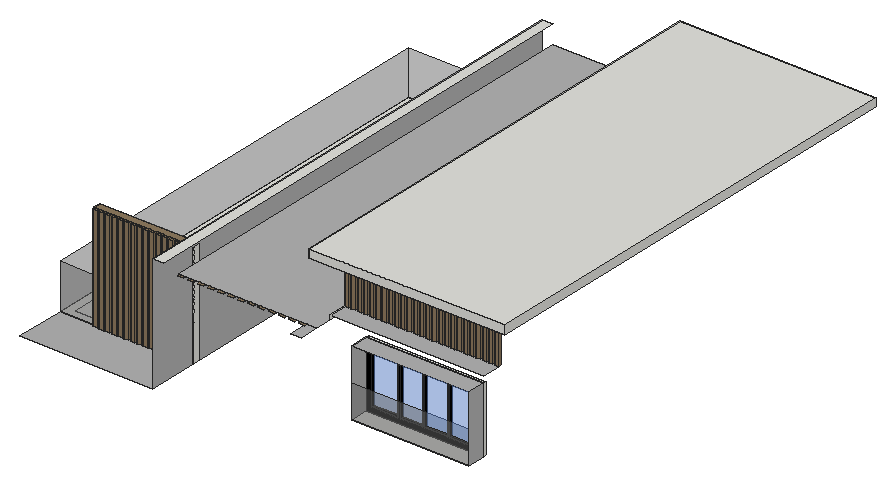
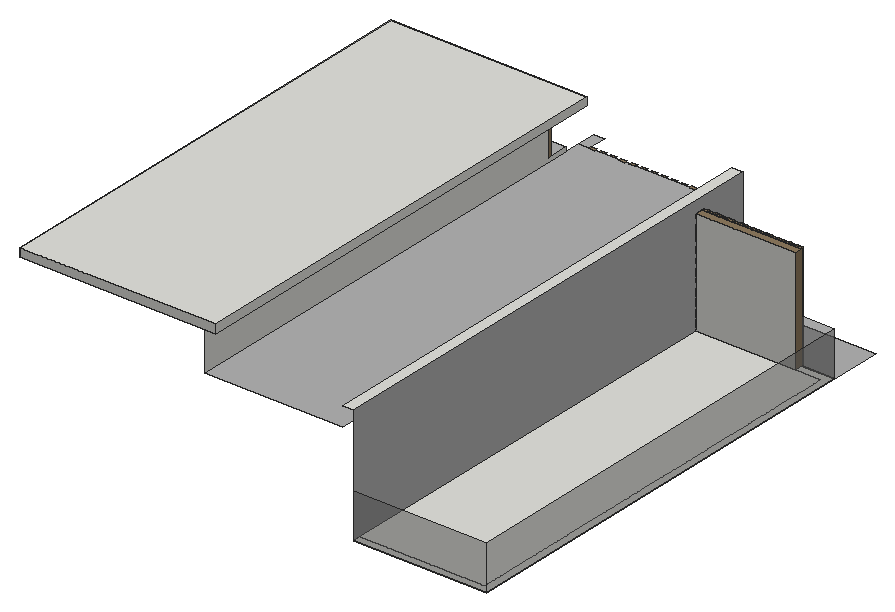
# SketchUp Ruby script. Lengths in inches.
U = 1.inch
M = Sketchup.active_model
def pt(a) = Geom::Point3d.new(a.map { |v| v * U })
def face(e, loops, mat)
  f = e.add_face(loops[0].map { |a| pt(a) })
  loops[1..].each { |l| e.add_face(l.map { |a| pt(a) }).erase! }
  f.material = f.back_material = mat if mat
  f
end
# faces: each face lists its corners as indices into pts; further lists are holes
def faces(e, pts, list, mat = nil) = list.each { |f| face(e, (f[0].is_a?(Array) ? f : [f]).map { |l| l.map { |i| pts[i] } }, mat) }
# xy, xz, yz: faces in a plane at the given z, y or x. An outline is a flat list of corners, or four numbers for a rectangle; further outlines are holes
def ring(l) = l.size == 4 ? [[l[0], l[1]], [l[2], l[1]], [l[2], l[3]], [l[0], l[3]]] : l.each_slice(2).to_a
def flat(e, list, mat, &to3) = list.each { |f| face(e, (f[0].is_a?(Array) ? f : [f]).map { |l| ring(l).map { |u, v| to3.(u, v) } }, mat) }
def xy(e, z, list, mat = nil) = flat(e, list, mat) { |x, y| [x, y, z] }
def xz(e, y, list, mat = nil) = flat(e, list, mat) { |x, z| [x, y, z] }
def yz(e, x, list, mat = nil) = flat(e, list, mat) { |y, z| [x, y, z] }
def lines(e, pts, list) = list.each { |a, b| e.add_line(pt(pts[a]), pt(pts[b])) }
# prism: a flat outline (further loops are holes) pulled along v
def prism(e, loops, v, mat = nil)
  f = face(e, loops, mat); d = Geom::Vector3d.new(v.map { |x| x * U })
  f.pushpull(f.normal.samedirection?(d) ? d.length : -d.length)
end
def box(e, o, s, mat = nil) = prism(e, [[o, [o[0] + s[0], o[1], o[2]], [o[0] + s[0], o[1] + s[1], o[2]], [o[0], o[1] + s[1], o[2]]]], [0, 0, s[2]], mat)
def at(x, y, z, deg = 0) = Geom::Transformation.translation(pt([x, y, z])) * Geom::Transformation.rotation(ORIGIN, Z_AXIS, deg.degrees)
def axes(o, x, y, z) = Geom::Transformation.new([*x, 0, *y, 0, *z, 0, *pt(o).to_a, 1])
def part(name) = M.definitions.add(name)
# library, detail: a bought-in or finely detailed component or shape, given as its bounding box
def library(name, o, s) = part(name).tap { |d| box(d.entities, o, s) }
def detail(e, o, s) = box(e.add_group.entities, o, s)
def put(e, d, t, mat = nil) = e.add_instance(d, t).tap { |i| i.material = mat if mat }
def group(e, t, mat = nil) = e.add_group.tap { |g| g.transformation = t; g.material = mat if mat }.entities
root = M.entities
M.materials.add("Niraj_Hair_Gray").color = [178, 178, 178]
M.materials.add("[0035_Tan]").color = [142, 122, 95]
M.materials.add("[0137_Black]").color = [0, 0, 0]
M.materials.add("[Translucent Glass Blue]").color = [100, 149, 237]
M.materials["[Translucent Glass Blue]"].alpha = 0.5
M.materials.add("[Translucent Glass Gray]").color = [128, 128, 128]
M.materials["[Translucent Glass Gray]"].alpha = 0.5
xy(root,261.125,[[39.27,322.73,44.8,325.73],[46.45,322.73,51.99,325.73],[53.64,322.73,59.17,325.73],[60.83,322.73,66.36,325.73],[68.02,322.73,73.55,325.73],
  [75.2,322.73,80.74,325.73],[82.39,322.73,87.92,325.73],[89.58,322.73,95.11,325.73],[96.77,322.73,102.3,325.73],[103.95,322.73,109.49,325.73],
  [111.14,322.73,116.67,325.73],[118.33,322.73,123.86,325.73],[125.52,322.73,131.05,325.73],[132.7,322.73,138.24,325.73],[139.89,322.73,145.42,325.73],
  [147.08,322.73,152.61,325.73],[0,325.73,38.3125,325.73,38.3125,334.73,9,334.73,9,814.73,151.88,814.73,151.88,823.73,0,823.73],[38.3125,325.73,152.61,334.73],[9,334.73,152.61,334.73,152.61,823.73,151.88,823.73,151.88,814.73,9,814.73]])
xy(root,261.125,[[0,267.73,152.61,267.73,152.61,322.73,147.08,322.73,147.08,325.73,145.42,325.73,145.42,322.73,139.89,322.73,139.89,325.73,138.24,325.73,138.24,322.73,132.7,322.73,132.7,325.73,131.05,325.73,131.05,322.73,125.52,322.73,125.52,325.73,123.86,325.73,123.86,322.73,118.33,322.73,118.33,325.73,116.67,325.73,116.67,322.73,111.14,322.73,111.14,325.73,109.49,325.73,109.49,322.73,103.95,322.73,103.95,325.73,102.3,325.73,102.3,322.73,96.77,322.73,96.77,325.73,95.11,325.73,95.11,322.73,89.58,322.73,89.58,325.73,87.92,325.73,87.92,322.73,82.39,322.73,82.39,325.73,80.74,325.73,80.74,322.73,75.2,322.73,75.2,325.73,73.55,325.73,73.55,322.73,68.02,322.73,68.02,325.73,66.36,325.73,66.36,322.73,60.83,322.73,60.83,325.73,59.17,325.73,59.17,322.73,53.64,322.73,53.64,325.73,51.99,325.73,51.99,322.73,46.45,322.73,46.45,325.73,44.8,325.73,44.8,322.73,39.27,322.73,39.27,325.73,0,325.73]],"Niraj_Hair_Gray")
xy(root,279.54,[[346.71,308.48,480.7,329.48],[346.71,329.48,480.7,332.48]])
xy(root,285.54,[[352.71,329.48,383.35,332.48],[386.35,329.48,411.04,332.48],[414.04,329.48,439.47,332.48],[442.47,329.48,474.7,332.48]],"[0137_Black]")
xy(root,349.07,[[352.71,329.48,383.35,332.48],[386.35,329.48,411.04,332.48],[414.04,329.48,439.47,332.48],[442.47,329.48,474.7,332.48]],"[0137_Black]")
xy(root,355.07,[[346.71,329.48,480.7,332.48]])
xy(root,355.07,[[346.71,308.48,480.7,329.48]],"Niraj_Hair_Gray")
xy(root,372.875,[[310.3125,267.73,322.3125,289.73],[164.61,289.73,322.3125,823.73]],"Niraj_Hair_Gray")
xy(root,372.875,[[165.47,286.73,172.3125,289.73],[176.97,286.73,183.8125,289.73],[188.47,286.73,195.3125,289.73],[199.97,286.73,206.8125,289.73],[211.47,286.73,218.3125,289.73],
  [222.97,286.73,229.8125,289.73],[234.47,286.73,241.3125,289.73],[245.97,286.73,252.8125,289.73],[257.47,286.73,264.3125,289.73],[268.97,286.73,275.8125,289.73],
  [280.47,286.73,287.3125,289.73],[291.97,286.73,298.8125,289.73],[303.47,286.73,310.3125,289.73]],"[0035_Tan]")
xy(root,377.94,[[322.3125,329.48,327.2,332.48],[329.4375,329.48,334.33,332.48],[336.5625,329.48,341.45,332.48],[343.6875,329.48,348.58,332.48],[350.8125,329.48,355.7,332.48],
  [357.9375,329.48,362.83,332.48],[365.0625,329.48,369.95,332.48],[372.1875,329.48,377.08,332.48],[379.3125,329.48,384.2,332.48],[386.4375,329.48,391.33,332.48],
  [393.5625,329.48,398.45,332.48],[400.6875,329.48,405.58,332.48],[407.8125,329.48,412.7,332.48],[414.9375,329.48,419.83,332.48],[422.0625,329.48,426.95,332.48],
  [429.1875,329.48,434.08,332.48],[436.375,329.48,441.27,332.48],[443.5625,329.48,448.45,332.48],[450.75,329.48,455.64,332.48],[457.9375,329.48,462.83,332.48],
  [465.125,329.48,470.02,332.48],[472.3125,329.48,477.2,332.48],[479.5,329.48,484.39,332.48],[486.6875,329.48,491.58,332.48],[493.875,329.48,498,332.48]])
xy(root,377.94,[[322.3125,308.48,498,308.48,498,329.48,493.875,329.48,493.875,332.48,491.58,332.48,491.58,329.48,486.6875,329.48,486.6875,332.48,484.39,332.48,484.39,329.48,479.5,329.48,479.5,332.48,477.2,332.48,477.2,329.48,472.3125,329.48,472.3125,332.48,470.02,332.48,470.02,329.48,465.125,329.48,465.125,332.48,462.83,332.48,462.83,329.48,457.9375,329.48,457.9375,332.48,455.64,332.48,455.64,329.48,450.75,329.48,450.75,332.48,448.45,332.48,448.45,329.48,443.5625,329.48,443.5625,332.48,441.27,332.48,441.27,329.48,436.375,329.48,436.375,332.48,434.08,332.48,434.08,329.48,429.1875,329.48,429.1875,332.48,426.95,332.48,426.95,329.48,422.0625,329.48,422.0625,332.48,419.83,332.48,419.83,329.48,414.9375,329.48,414.9375,332.48,412.7,332.48,412.7,329.48,407.8125,329.48,407.8125,332.48,405.58,332.48,405.58,329.48,400.6875,329.48,400.6875,332.48,398.45,332.48,398.45,329.48,393.5625,329.48,393.5625,332.48,391.33,332.48,391.33,329.48,386.4375,329.48,386.4375,332.48,384.2,332.48,384.2,329.48,379.3125,329.48,379.3125,332.48,377.08,332.48,377.08,329.48,372.1875,329.48,372.1875,332.48,369.95,332.48,369.95,329.48,365.0625,329.48,365.0625,332.48,362.83,332.48,362.83,329.48,357.9375,329.48,357.9375,332.48,355.7,332.48,355.7,329.48,350.8125,329.48,350.8125,332.48,348.58,332.48,348.58,329.48,343.6875,329.48,343.6875,332.48,341.45,332.48,341.45,329.48,336.5625,329.48,336.5625,332.48,334.33,332.48,334.33,329.48,329.4375,329.48,329.4375,332.48,327.2,332.48,327.2,329.48,322.3125,329.48]],"Niraj_Hair_Gray")
xy(root,381.125,[[39.27,322.73,44.8,325.73],[46.45,322.73,51.99,325.73],[53.64,322.73,59.17,325.73],[60.83,322.73,66.36,325.73],[68.02,322.73,73.55,325.73],
  [75.2,322.73,80.74,325.73],[82.39,322.73,87.92,325.73],[89.58,322.73,95.11,325.73],[96.77,322.73,102.3,325.73],[103.95,322.73,109.49,325.73],
  [111.14,322.73,116.67,325.73],[118.33,322.73,123.86,325.73],[125.52,322.73,131.05,325.73],[132.7,322.73,138.24,325.73],[139.89,322.73,145.42,325.73],
  [147.08,322.73,152.61,325.73],[38.3125,325.73,152.61,334.73]],"[0035_Tan]")
xy(root,394.4375,[[152.61,267.73,164.61,823.73]])
xy(root,428.22,[[[298.3125,308.48,522,838.73],[322.3125,329.48,327.2,329.48,327.2,332.48,329.4375,332.48,329.4375,329.48,334.33,329.48,334.33,332.48,336.5625,332.48,336.5625,329.48,341.45,329.48,341.45,332.48,343.6875,332.48,343.6875,329.48,348.58,329.48,348.58,332.48,350.8125,332.48,350.8125,329.48,355.7,329.48,355.7,332.48,357.9375,332.48,357.9375,329.48,362.83,329.48,362.83,332.48,365.0625,332.48,365.0625,329.48,369.95,329.48,369.95,332.48,372.1875,332.48,372.1875,329.48,377.08,329.48,377.08,332.48,379.3125,332.48,379.3125,329.48,384.2,329.48,384.2,332.48,386.4375,332.48,386.4375,329.48,391.33,329.48,391.33,332.48,393.5625,332.48,393.5625,329.48,398.45,329.48,398.45,332.48,400.6875,332.48,400.6875,329.48,405.58,329.48,405.58,332.48,407.8125,332.48,407.8125,329.48,412.7,329.48,412.7,332.48,414.9375,332.48,414.9375,329.48,419.83,329.48,419.83,332.48,422.0625,332.48,422.0625,329.48,426.95,329.48,426.95,332.48,429.1875,332.48,429.1875,329.48,434.08,329.48,434.08,332.48,436.375,332.48,436.375,329.48,441.27,329.48,441.27,332.48,443.5625,332.48,443.5625,329.48,448.45,329.48,448.45,332.48,450.75,332.48,450.75,329.48,455.64,329.48,455.64,332.48,457.9375,332.48,457.9375,329.48,462.83,329.48,462.83,332.48,465.125,332.48,465.125,329.48,470.02,329.48,470.02,332.48,472.3125,332.48,472.3125,329.48,477.2,329.48,477.2,332.48,479.5,332.48,479.5,329.48,484.39,329.48,484.39,332.48,486.6875,332.48,486.6875,329.48,491.58,329.48,491.58,332.48,493.875,332.48,493.875,329.48,498,329.48,498,823.73,322.3125,823.73]],[322.3125,329.48,327.2,332.48],[329.4375,329.48,334.33,332.48],[336.5625,329.48,341.45,332.48],[343.6875,329.48,348.58,332.48],
  [350.8125,329.48,355.7,332.48],[357.9375,329.48,362.83,332.48],[365.0625,329.48,369.95,332.48],[372.1875,329.48,377.08,332.48],[379.3125,329.48,384.2,332.48],
  [386.4375,329.48,391.33,332.48],[393.5625,329.48,398.45,332.48],[400.6875,329.48,405.58,332.48],[407.8125,329.48,412.7,332.48],[414.9375,329.48,419.83,332.48],
  [422.0625,329.48,426.95,332.48],[429.1875,329.48,434.08,332.48],[436.375,329.48,441.27,332.48],[443.5625,329.48,448.45,332.48],[450.75,329.48,455.64,332.48],
  [457.9375,329.48,462.83,332.48],[465.125,329.48,470.02,332.48],[472.3125,329.48,477.2,332.48],[479.5,329.48,484.39,332.48],[486.6875,329.48,491.58,332.48],
  [493.875,329.48,498,332.48],[322.3125,332.48,498,823.73]])
xy(root,437.94,[[298.3125,308.48,522,838.73]])
xz(root,308.48,[[298.3125,428.22,522,437.94]])
xz(root,308.48,[[346.71,279.54,480.7,317.3]],"[Translucent Glass Gray]")
xz(root,322.73,[[39.27,261.125,44.8,381.125],[46.45,261.125,51.99,381.125],[53.64,261.125,59.17,381.125],[60.83,261.125,66.36,381.125],[68.02,261.125,73.55,381.125],
  [75.2,261.125,80.74,381.125],[82.39,261.125,87.92,381.125],[89.58,261.125,95.11,381.125],[96.77,261.125,102.3,381.125],[103.95,261.125,109.49,381.125],
  [111.14,261.125,116.67,381.125],[118.33,261.125,123.86,381.125],[125.52,261.125,131.05,381.125],[132.7,261.125,138.24,381.125],[139.89,261.125,145.42,381.125],
  [147.08,261.125,152.61,381.125]],"[0035_Tan]")
xz(root,325.73,[[39.27,261.125,44.8,381.125],[46.45,261.125,51.99,381.125],[53.64,261.125,59.17,381.125],[60.83,261.125,66.36,381.125],[68.02,261.125,73.55,381.125],
  [75.2,261.125,80.74,381.125],[82.39,261.125,87.92,381.125],[89.58,261.125,95.11,381.125],[96.77,261.125,102.3,381.125],[103.95,261.125,109.49,381.125],
  [111.14,261.125,116.67,381.125],[118.33,261.125,123.86,381.125],[125.52,261.125,131.05,381.125],[132.7,261.125,138.24,381.125],[139.89,261.125,145.42,381.125],
  [147.08,261.125,152.61,381.125]])
xz(root,325.73,[[38.3125,261.125,39.27,381.125],[44.8,261.125,46.45,381.125],[51.99,261.125,53.64,381.125],[59.17,261.125,60.83,381.125],[66.36,261.125,68.02,381.125],
  [73.55,261.125,75.2,381.125],[80.74,261.125,82.39,381.125],[87.92,261.125,89.58,381.125],[95.11,261.125,96.77,381.125],[102.3,261.125,103.95,381.125],
  [109.49,261.125,111.14,381.125],[116.67,261.125,118.33,381.125],[123.86,261.125,125.52,381.125],[131.05,261.125,132.7,381.125],[138.24,261.125,139.89,381.125],
  [145.42,261.125,147.08,381.125]],"[0035_Tan]")
xz(root,325.73,[[0,261.125,38.3125,312.39]],"[Translucent Glass Gray]")
xz(root,329.48,[[322.3125,377.94,327.2,428.22],[329.4375,377.94,334.33,428.22],[336.5625,377.94,341.45,428.22],[343.6875,377.94,348.58,428.22],[350.8125,377.94,355.7,428.22],
  [357.9375,377.94,362.83,428.22],[365.0625,377.94,369.95,428.22],[372.1875,377.94,377.08,428.22],[379.3125,377.94,384.2,428.22],[386.4375,377.94,391.33,428.22],
  [393.5625,377.94,398.45,428.22],[400.6875,377.94,405.58,428.22],[407.8125,377.94,412.7,428.22],[414.9375,377.94,419.83,428.22],[422.0625,377.94,426.95,428.22],
  [429.1875,377.94,434.08,428.22],[436.375,377.94,441.27,428.22],[443.5625,377.94,448.45,428.22],[450.75,377.94,455.64,428.22],[457.9375,377.94,462.83,428.22],
  [465.125,377.94,470.02,428.22],[472.3125,377.94,477.2,428.22],[479.5,377.94,484.39,428.22],[486.6875,377.94,491.58,428.22],[493.875,377.94,498,428.22]],"[0035_Tan]")
xz(root,329.48,[[[346.71,279.54,480.7,355.07],[442.47,285.54,474.7,349.07],[352.71,285.54,383.35,349.07],[414.04,285.54,439.47,349.07],[386.35,285.54,411.04,349.07]]],"[0137_Black]")
xz(root,332.48,[[322.3125,377.94,327.2,428.22],[329.4375,377.94,334.33,428.22],[336.5625,377.94,341.45,428.22],[343.6875,377.94,348.58,428.22],[350.8125,377.94,355.7,428.22],
  [357.9375,377.94,362.83,428.22],[365.0625,377.94,369.95,428.22],[372.1875,377.94,377.08,428.22],[379.3125,377.94,384.2,428.22],[386.4375,377.94,391.33,428.22],
  [393.5625,377.94,398.45,428.22],[400.6875,377.94,405.58,428.22],[407.8125,377.94,412.7,428.22],[414.9375,377.94,419.83,428.22],[422.0625,377.94,426.95,428.22],
  [429.1875,377.94,434.08,428.22],[436.375,377.94,441.27,428.22],[443.5625,377.94,448.45,428.22],[450.75,377.94,455.64,428.22],[457.9375,377.94,462.83,428.22],
  [465.125,377.94,470.02,428.22],[472.3125,377.94,477.2,428.22],[479.5,377.94,484.39,428.22],[486.6875,377.94,491.58,428.22],[493.875,377.94,498,428.22]])
xz(root,332.48,[[327.2,377.94,329.4375,428.22],[334.33,377.94,336.5625,428.22],[341.45,377.94,343.6875,428.22],[348.58,377.94,350.8125,428.22],[355.7,377.94,357.9375,428.22],
  [362.83,377.94,365.0625,428.22],[369.95,377.94,372.1875,428.22],[377.08,377.94,379.3125,428.22],[384.2,377.94,386.4375,428.22],[391.33,377.94,393.5625,428.22],
  [398.45,377.94,400.6875,428.22],[405.58,377.94,407.8125,428.22],[412.7,377.94,414.9375,428.22],[419.83,377.94,422.0625,428.22],[426.95,377.94,429.1875,428.22],
  [434.08,377.94,436.375,428.22],[441.27,377.94,443.5625,428.22],[448.45,377.94,450.75,428.22],[455.64,377.94,457.9375,428.22],[462.83,377.94,465.125,428.22],
  [470.02,377.94,472.3125,428.22],[477.2,377.94,479.5,428.22],[484.39,377.94,486.6875,428.22],[491.58,377.94,493.875,428.22]],"[0035_Tan]")
xz(root,332.48,[[352.71,285.54,383.35,349.07],[386.35,285.54,411.04,349.07],[414.04,285.54,439.47,349.07],[442.47,285.54,474.7,349.07]],"[Translucent Glass Blue]")
xz(root,334.73,[[38.3125,261.125,151.88,381.125],[151.88,261.125,152.61,381.125]])
xz(root,823.73,[[0,261.125,151.88,312.39]],"[Translucent Glass Gray]")
xz(root,838.73,[[298.3125,428.22,522,437.94]])
yz(root,0,[[325.73,261.125,823.73,312.39]],"[Translucent Glass Gray]")
yz(root,38.3125,[[325.73,261.125,334.73,381.125]],"[0035_Tan]")
yz(root,39.27,[[322.73,261.125,325.73,381.125]],"[0035_Tan]")
yz(root,44.8,[[322.73,261.125,325.73,381.125]],"[0035_Tan]")
yz(root,46.45,[[322.73,261.125,325.73,381.125]],"[0035_Tan]")
yz(root,51.99,[[322.73,261.125,325.73,381.125]],"[0035_Tan]")
yz(root,53.64,[[322.73,261.125,325.73,381.125]],"[0035_Tan]")
yz(root,59.17,[[322.73,261.125,325.73,381.125]],"[0035_Tan]")
yz(root,60.83,[[322.73,261.125,325.73,381.125]],"[0035_Tan]")
yz(root,66.36,[[322.73,261.125,325.73,381.125]],"[0035_Tan]")
yz(root,68.02,[[322.73,261.125,325.73,381.125]],"[0035_Tan]")
yz(root,73.55,[[322.73,261.125,325.73,381.125]],"[0035_Tan]")
yz(root,75.2,[[322.73,261.125,325.73,381.125]],"[0035_Tan]")
yz(root,80.74,[[322.73,261.125,325.73,381.125]],"[0035_Tan]")
yz(root,82.39,[[322.73,261.125,325.73,381.125]],"[0035_Tan]")
yz(root,87.92,[[322.73,261.125,325.73,381.125]],"[0035_Tan]")
yz(root,89.58,[[322.73,261.125,325.73,381.125]],"[0035_Tan]")
yz(root,95.11,[[322.73,261.125,325.73,381.125]],"[0035_Tan]")
yz(root,96.77,[[322.73,261.125,325.73,381.125]],"[0035_Tan]")
yz(root,102.3,[[322.73,261.125,325.73,381.125]],"[0035_Tan]")
yz(root,103.95,[[322.73,261.125,325.73,381.125]],"[0035_Tan]")
yz(root,109.49,[[322.73,261.125,325.73,381.125]],"[0035_Tan]")
yz(root,111.14,[[322.73,261.125,325.73,381.125]],"[0035_Tan]")
yz(root,116.67,[[322.73,261.125,325.73,381.125]],"[0035_Tan]")
yz(root,118.33,[[322.73,261.125,325.73,381.125]],"[0035_Tan]")
yz(root,123.86,[[322.73,261.125,325.73,381.125]],"[0035_Tan]")
yz(root,125.52,[[322.73,261.125,325.73,381.125]],"[0035_Tan]")
yz(root,131.05,[[322.73,261.125,325.73,381.125]],"[0035_Tan]")
yz(root,132.7,[[322.73,261.125,325.73,381.125]],"[0035_Tan]")
yz(root,138.24,[[322.73,261.125,325.73,381.125]],"[0035_Tan]")
yz(root,139.89,[[322.73,261.125,325.73,381.125]],"[0035_Tan]")
yz(root,145.42,[[322.73,261.125,325.73,381.125]],"[0035_Tan]")
yz(root,147.08,[[322.73,261.125,325.73,381.125]],"[0035_Tan]")
yz(root,152.61,[[322.73,261.125,325.73,381.125],[325.73,261.125,334.73,381.125]])
yz(root,152.61,[[267.73,261.125,267.73,394.4375,823.73,394.4375,823.73,261.125,334.73,261.125,334.73,381.125,322.73,381.125,322.73,261.125]],"Niraj_Hair_Gray")
yz(root,298.3125,[[308.48,428.22,838.73,437.94]])
yz(root,322.3125,[[308.48,372.875,308.48,377.94,332.48,377.94,332.48,428.22,823.73,428.22,823.73,372.875]])
yz(root,322.3125,[[329.48,377.94,332.48,428.22]],"[0035_Tan]")
yz(root,327.2,[[329.48,377.94,332.48,428.22]],"[0035_Tan]")
yz(root,329.4375,[[329.48,377.94,332.48,428.22]],"[0035_Tan]")
yz(root,334.33,[[329.48,377.94,332.48,428.22]],"[0035_Tan]")
yz(root,336.5625,[[329.48,377.94,332.48,428.22]],"[0035_Tan]")
yz(root,341.45,[[329.48,377.94,332.48,428.22]],"[0035_Tan]")
yz(root,343.6875,[[329.48,377.94,332.48,428.22]],"[0035_Tan]")
yz(root,346.71,[[329.48,279.54,332.48,355.07]])
yz(root,346.71,[[308.48,279.54,329.48,355.07]],"Niraj_Hair_Gray")
yz(root,348.58,[[329.48,377.94,332.48,428.22]],"[0035_Tan]")
yz(root,350.8125,[[329.48,377.94,332.48,428.22]],"[0035_Tan]")
yz(root,352.71,[[329.48,285.54,332.48,349.07]],"[0137_Black]")
yz(root,355.7,[[329.48,377.94,332.48,428.22]],"[0035_Tan]")
yz(root,357.9375,[[329.48,377.94,332.48,428.22]],"[0035_Tan]")
yz(root,362.83,[[329.48,377.94,332.48,428.22]],"[0035_Tan]")
yz(root,365.0625,[[329.48,377.94,332.48,428.22]],"[0035_Tan]")
yz(root,369.95,[[329.48,377.94,332.48,428.22]],"[0035_Tan]")
yz(root,372.1875,[[329.48,377.94,332.48,428.22]],"[0035_Tan]")
yz(root,377.08,[[329.48,377.94,332.48,428.22]],"[0035_Tan]")
yz(root,379.3125,[[329.48,377.94,332.48,428.22]],"[0035_Tan]")
yz(root,383.35,[[329.48,285.54,332.48,349.07]],"[0137_Black]")
yz(root,384.2,[[329.48,377.94,332.48,428.22]],"[0035_Tan]")
yz(root,386.35,[[329.48,285.54,332.48,349.07]],"[0137_Black]")
yz(root,386.4375,[[329.48,377.94,332.48,428.22]],"[0035_Tan]")
yz(root,391.33,[[329.48,377.94,332.48,428.22]],"[0035_Tan]")
yz(root,393.5625,[[329.48,377.94,332.48,428.22]],"[0035_Tan]")
yz(root,398.45,[[329.48,377.94,332.48,428.22]],"[0035_Tan]")
yz(root,400.6875,[[329.48,377.94,332.48,428.22]],"[0035_Tan]")
yz(root,405.58,[[329.48,377.94,332.48,428.22]],"[0035_Tan]")
yz(root,407.8125,[[329.48,377.94,332.48,428.22]],"[0035_Tan]")
yz(root,411.04,[[329.48,285.54,332.48,349.07]],"[0137_Black]")
yz(root,412.7,[[329.48,377.94,332.48,428.22]],"[0035_Tan]")
yz(root,414.04,[[329.48,285.54,332.48,349.07]],"[0137_Black]")
yz(root,414.9375,[[329.48,377.94,332.48,428.22]],"[0035_Tan]")
yz(root,419.83,[[329.48,377.94,332.48,428.22]],"[0035_Tan]")
yz(root,422.0625,[[329.48,377.94,332.48,428.22]],"[0035_Tan]")
yz(root,426.95,[[329.48,377.94,332.48,428.22]],"[0035_Tan]")
yz(root,429.1875,[[329.48,377.94,332.48,428.22]],"[0035_Tan]")
yz(root,434.08,[[329.48,377.94,332.48,428.22]],"[0035_Tan]")
yz(root,436.375,[[329.48,377.94,332.48,428.22]],"[0035_Tan]")
yz(root,439.47,[[329.48,285.54,332.48,349.07]],"[0137_Black]")
yz(root,441.27,[[329.48,377.94,332.48,428.22]],"[0035_Tan]")
yz(root,442.47,[[329.48,285.54,332.48,349.07]],"[0137_Black]")
yz(root,443.5625,[[329.48,377.94,332.48,428.22]],"[0035_Tan]")
yz(root,448.45,[[329.48,377.94,332.48,428.22]],"[0035_Tan]")
yz(root,450.75,[[329.48,377.94,332.48,428.22]],"[0035_Tan]")
yz(root,455.64,[[329.48,377.94,332.48,428.22]],"[0035_Tan]")
yz(root,457.9375,[[329.48,377.94,332.48,428.22]],"[0035_Tan]")
yz(root,462.83,[[329.48,377.94,332.48,428.22]],"[0035_Tan]")
yz(root,465.125,[[329.48,377.94,332.48,428.22]],"[0035_Tan]")
yz(root,470.02,[[329.48,377.94,332.48,428.22]],"[0035_Tan]")
yz(root,472.3125,[[329.48,377.94,332.48,428.22]],"[0035_Tan]")
yz(root,474.7,[[329.48,285.54,332.48,349.07]],"[0137_Black]")
yz(root,477.2,[[329.48,377.94,332.48,428.22]],"[0035_Tan]")
yz(root,479.5,[[329.48,377.94,332.48,428.22]],"[0035_Tan]")
yz(root,480.7,[[329.48,279.54,332.48,355.07]])
yz(root,480.7,[[308.48,279.54,329.48,355.07]],"Niraj_Hair_Gray")
yz(root,484.39,[[329.48,377.94,332.48,428.22]],"[0035_Tan]")
yz(root,486.6875,[[329.48,377.94,332.48,428.22]],"[0035_Tan]")
yz(root,491.58,[[329.48,377.94,332.48,428.22]],"[0035_Tan]")
yz(root,493.875,[[329.48,377.94,332.48,428.22]],"[0035_Tan]")
yz(root,498,[[329.48,377.94,332.48,428.22]],"[0035_Tan]")
yz(root,522,[[308.48,428.22,838.73,437.94]])
